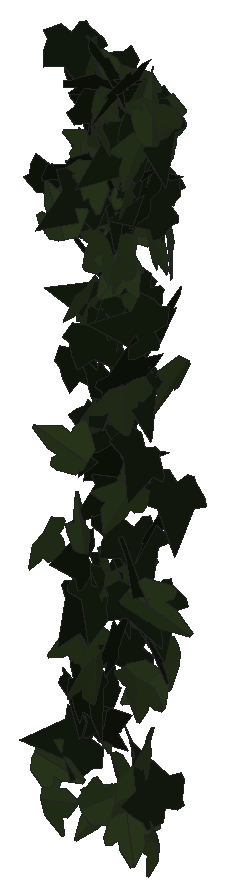
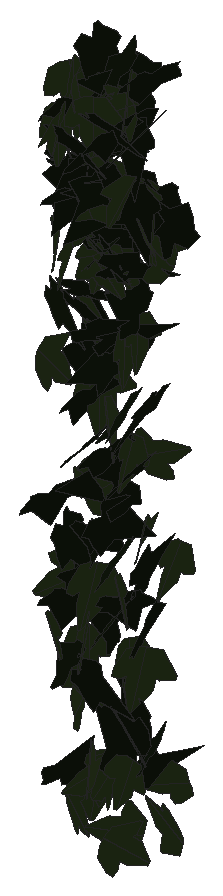
# SketchUp Ruby script. Lengths in inches.
U = 1.inch
M = Sketchup.active_model
def pt(a) = Geom::Point3d.new(a.map { |v| v * U })
def face(e, loops, mat)
  f = e.add_face(loops[0].map { |a| pt(a) })
  loops[1..].each { |l| e.add_face(l.map { |a| pt(a) }).erase! }
  f.material = f.back_material = mat if mat
  f
end
# faces: each face lists its corners as indices into pts; further lists are holes
def faces(e, pts, list, mat = nil) = list.each { |f| face(e, (f[0].is_a?(Array) ? f : [f]).map { |l| l.map { |i| pts[i] } }, mat) }
# xy, xz, yz: faces in a plane at the given z, y or x. An outline is a flat list of corners, or four numbers for a rectangle; further outlines are holes
def ring(l) = l.size == 4 ? [[l[0], l[1]], [l[2], l[1]], [l[2], l[3]], [l[0], l[3]]] : l.each_slice(2).to_a
def flat(e, list, mat, &to3) = list.each { |f| face(e, (f[0].is_a?(Array) ? f : [f]).map { |l| ring(l).map { |u, v| to3.(u, v) } }, mat) }
def xy(e, z, list, mat = nil) = flat(e, list, mat) { |x, y| [x, y, z] }
def xz(e, y, list, mat = nil) = flat(e, list, mat) { |x, z| [x, y, z] }
def yz(e, x, list, mat = nil) = flat(e, list, mat) { |y, z| [x, y, z] }
def lines(e, pts, list) = list.each { |a, b| e.add_line(pt(pts[a]), pt(pts[b])) }
# prism: a flat outline (further loops are holes) pulled along v
def prism(e, loops, v, mat = nil)
  f = face(e, loops, mat); d = Geom::Vector3d.new(v.map { |x| x * U })
  f.pushpull(f.normal.samedirection?(d) ? d.length : -d.length)
end
def box(e, o, s, mat = nil) = prism(e, [[o, [o[0] + s[0], o[1], o[2]], [o[0] + s[0], o[1] + s[1], o[2]], [o[0], o[1] + s[1], o[2]]]], [0, 0, s[2]], mat)
def at(x, y, z, deg = 0) = Geom::Transformation.translation(pt([x, y, z])) * Geom::Transformation.rotation(ORIGIN, Z_AXIS, deg.degrees)
def axes(o, x, y, z) = Geom::Transformation.new([*x, 0, *y, 0, *z, 0, *pt(o).to_a, 1])
def part(name) = M.definitions.add(name)
# library, detail: a bought-in or finely detailed component or shape, given as its bounding box
def library(name, o, s) = part(name).tap { |d| box(d.entities, o, s) }
def detail(e, o, s) = box(e.add_group.entities, o, s)
def put(e, d, t, mat = nil) = e.add_instance(d, t).tap { |i| i.material = mat if mat }
def group(e, t, mat = nil) = e.add_group.tap { |g| g.transformation = t; g.material = mat if mat }.entities
root = M.entities
M.materials.add("efeu1").color = [18, 25, 13]
M.materials.add("efeu2").color = [43, 57, 29]
c1 = part("ivyleaf_10")
p = [[0,0.5,-0.03],[-0.0625,2.02,-0.43],[-0.19,2.01,-0.46],[-0.54,1.05,-0.29],[-0.52,0.625,-0.18],[-0.83,0.76,-0.28],
  [-1.16,0.64,-0.33],[-1.15,0.33,-0.24],[-0.77,-0.39,0.02],[-0.3,-0.51,0.16],[0.04,-0.48,0.23],[-0.02,2.01,-0.4375],
  [-0.06,2.01,-0.43],[0.04,-0.49,0.23],[0.67,-0.49,0.14],[1.38,0.36,-0.2],[1.375,0.51,-0.24],[0.81,0.65,-0.19],
  [0.62,0.59,-0.15],[0.6,1.09,-0.28],[0.5,1.23,-0.31]]
faces(c1.entities,p,[[0,1,2,3,4,5,6,7,8,9,10],[11,12,0,13,14,15,16,17,18,19,20]],"efeu2")
c2 = part("ivyleaf_9")
p = [[1.54,2.16,1.25],[1.36,2.04,1.19],[-0.21,0.99,0.68],[-0.71,1.11,0.82],[-0.85,0.86,0.67],[-0.8,0.17,0.21],
  [-0.9,-0.01,0.1],[-0.67,-0.16,-0.02],[-0.08,-0.08,-0.05],[-0.03,-0.6,-0.4],[0.65,-0.88,-0.66],[0.83,-0.6,-0.49],
  [1.29,-0.42,-0.43],[1.8125,-0.07,-0.26],[1.21,0.44,0.15]]
faces(c2.entities,p,[[0,1,2,3,4,5,6,7,8,9,10,11,12,13,14]],"efeu1")
put(root,c1,axes([564.66,129.125,234.52],[0.19735,-0.83656,0.62727],[-0.15068,0.60893,0.85951],[-1.0347,-0.24823,-0.00552]))
put(root,c1,axes([564.375,130.51,235.96],[0.03234,-0.35529,-0.92496],[0.56311,-0.75489,0.30965],[-0.81529,-0.53548,0.17718]))
put(root,c2,axes([564.27,129.14,235.72],[-0.19011,-0.12223,1.03276],[0.96158,-0.42052,0.12724],[0.39609,0.96223,0.1868]))
put(root,c2,axes([564.42,130.8,241.61],[0.54974,-0.81143,-0.30196],[-0.02082,0.3452,-0.96552],[0.86555,0.52368,0.16856]))
put(root,c1,axes([564.88,128,219.98],[-0.06567,-0.82595,-0.60665],[0.21238,0.58373,-0.81773],[1.00255,-0.17776,0.13349]))
put(root,c2,axes([564.51,130.46,211.35],[0.19359,-0.71401,0.58022],[0.1566,-0.5587,-0.73978],[0.90661,0.24897,0.00389]))
put(root,c2,axes([565.46,130.25,237.87],[0.48085,0.32099,-0.82246],[-0.74029,-0.36372,-0.57477],[-0.48107,0.88054,0.0624]))
put(root,c1,axes([565.57,130.21,237.88],[-0.83667,-0.21288,0.52401],[-0.47896,-0.23101,-0.85858],[0.30084,-0.95981,0.09042]))
put(root,c2,axes([564.84,129.71,228.15],[0.54726,-0.5114,-0.69257],[-0.3479,0.61929,-0.7322],[0.78749,0.62898,0.15782]))
put(root,c1,axes([564.43,128.84,206.97],[0.2933,-0.21869,-1.04088],[0.88147,-0.55426,0.36483],[-0.59521,-0.92858,0.02738]))
put(root,c1,axes([564.55,128.25,209.1875],[0.2406,0.142,0.90249],[0.80852,0.40146,-0.27872],[-0.42539,0.84334,-0.01928]))
put(root,c2,axes([565.66,129.76,209.875],[-0.02498,-0.79926,-0.70561],[-0.01993,-0.70533,0.79965],[-1.06597,0.03192,0.00159]))
put(root,c2,axes([565.4,128.74,237.56],[0.57066,0.82522,-0.07792],[-0.05478,-0.05684,-1.00323],[-0.82708,0.57314,0.01269]))
put(root,c1,axes([565.62,128.08,234.97],[0.88424,0.19811,0.41243],[-0.40106,-0.09632,0.90614],[0.22021,-0.97092,-0.00574]))
put(root,c1,axes([565.42,130.67,210.56],[-0.91603,0.14415,-0.09368],[0.09303,-0.01147,-0.9273],[-0.14457,-0.92074,-0.00312]))
put(root,c2,axes([566.16,130.875,234.49],[-0.73813,-0.23105,0.65374],[-0.59549,-0.27786,-0.77057],[0.35517,-0.94604,0.06666]))
put(root,c2,axes([565.21,129.33,243.39],[0.06529,-0.94013,-0.42619],[0.07375,0.4302,-0.93768],[1.02959,0.0288,0.09419]))
put(root,c1,axes([566.28,128.26,224.28],[0.41224,0.27682,0.93431],[-0.85578,-0.38233,0.49088],[0.46604,-0.94694,0.07493]))
put(root,c1,axes([565.77,129.46,231.25],[0.01711,-0.9549,-0.29214],[0.03731,0.29259,-0.95418],[0.99789,0.00544,0.04069]))
put(root,c1,axes([565.8,129.15,214.99],[-0.68211,-0.81872,-0.27806],[0.18071,0.21137,-1.06562],[0.84555,-0.70563,0.00343]))
put(root,c1,axes([565.88,129.76,225.54],[0.00864,-0.791,-0.58161],[0.08915,0.57986,-0.7873],[0.97775,-0.04588,0.07692]))
put(root,c1,axes([565.74,130.1875,238.24],[0.09132,0.88481,0.46957],[0.01194,0.47053,-0.88892],[-1.00162,0.08628,0.03221]))
put(root,c2,axes([565.67,130.66,224.32],[-0.19662,-0.82672,0.54571],[0.00532,-0.55723,-0.84226],[0.99058,-0.16111,0.11284]))
put(root,c2,axes([565.15,130.36,232.42],[0.47835,-0.53882,0.69882],[0.45037,-0.53449,-0.7204],[0.75884,0.65687,-0.01296]))
put(root,c1,axes([565.98,130.1,230.75],[0.07186,-0.95686,-0.27886],[0.0528,0.28284,-0.95693],[0.99526,0.05408,0.0709]))
put(root,c2,axes([565.96,129.32,218.83],[-0.09449,-0.23298,0.97162],[-0.36011,-0.90242,-0.25141],[0.93201,-0.3723,0.00136]))
put(root,c1,axes([566.2,130.64,206.67],[-0.27259,-0.54875,0.84407],[-0.11609,-0.8515,-0.59107],[1.00006,-0.24842,0.16146]))
put(root,c2,axes([566.3,129.26,236.32],[-0.57538,-0.5983,0.55719],[-0.40314,-0.38512,-0.82985],[0.71127,-0.70228,-0.01961]))
put(root,c2,axes([566.3,129.15,240.3],[0.60577,0.21239,-0.79905],[-0.79349,-0.12896,-0.63584],[-0.23229,0.99439,0.0882]))
put(root,c2,axes([565.625,129.29,216.7],[0.32601,-0.31201,-1.00483],[0.75099,-0.66778,0.45101],[-0.73692,-0.81856,0.01508]))
put(root,c1,axes([566.59,128.95,237.2],[0.61229,-0.02497,-0.8142],[-0.8062,0.12723,-0.61017],[0.11661,1.01076,0.05669]))
put(root,c1,axes([566.23,129.35,242.62],[0.29267,-0.75201,-0.67991],[-0.0384,0.69894,-0.78959],[1.01307,0.24374,0.1665]))
put(root,c1,axes([566.42,128.37,220.19],[-0.2211,0.82835,-0.48441],[-0.18007,0.45246,0.8559],[0.94255,0.28075,0.04988]))
put(root,c2,axes([566.83,130.34,230.6],[-0.4043,-0.76048,-0.65377],[-0.30929,-0.57599,0.86127],[-0.95399,0.50904,-0.00217]))
put(root,c2,axes([566.9,129.33,211.84],[-0.44266,0.65901,0.74542],[-0.40501,0.62587,-0.79382],[-0.9088,-0.59991,-0.00931]))
put(root,c2,axes([566.1875,128.24,213.5],[0.5943,-0.36565,-0.72433],[-0.60709,0.39529,-0.69766],[0.53832,0.84946,0.01287]))
put(root,c2,axes([566.03,131.06,241.12],[0.01227,-1.00353,-0.14543],[-0.01055,0.14531,-1.00357],[1.01396,0.01365,-0.00868]))
put(root,c1,axes([566.74,129.5625,218.35],[0.3735,-0.46335,-0.72167],[-0.41284,0.5928,-0.59427],[0.75171,0.55579,0.0322]))
put(root,c1,axes([566.05,129.69,206.86],[-0.12735,-0.32235,0.95032],[0.3282,0.89188,0.3465],[-0.94832,0.35196,-0.0077]))
put(root,c2,axes([566.91,131.05,241.37],[-0.99688,0.00409,0.06429],[-0.0644,-0.08931,-0.99288],[0.00169,-0.99495,0.08939]))
put(root,c2,axes([566.76,130.97,235.79],[-0.78608,-0.49452,0.32912],[-0.20836,-0.28168,-0.92089],[0.55629,-0.8043,0.12015]))
put(root,c2,axes([566,129.4375,213.25],[-0.37797,-0.16034,-0.92484],[0.9199,0.13495,-0.39935],[0.18662,-0.98994,0.09536]))
put(root,c2,axes([565.99,130.84,217.66],[0.42607,-0.98165,0.06298],[0.02868,-0.05621,-1.07013],[0.98325,0.42702,0.00392]))
put(root,c2,axes([566.03,130.05,227.23],[0.59911,-0.76727,-0.08514],[-0.04238,0.07492,-0.97339],[0.77082,0.60048,0.01266]))
put(root,c1,axes([566,130.11,241.92],[-0.57607,0.12856,-0.81085],[0.69461,-0.45171,-0.5651],[-0.43764,-0.88617,0.17042]))
put(root,c1,axes([566.86,129.16,233.95],[0.79232,-0.30631,-0.63638],[-0.49482,0.44166,-0.82865],[0.50394,0.91525,0.18689]))
put(root,c2,axes([566.78,130.55,222.14],[-0.09942,0.03829,-0.96352],[0.16269,-0.95408,-0.0547],[-0.95046,-0.16732,0.09143]))
put(root,c2,axes([565.76,129.84,210.83],[0.96779,0.04784,-0.53455],[0.51249,0.24487,0.94976],[0.15934,-1.07815,0.19199]))
put(root,c1,axes([566.79,130.83,234.5],[0.81735,0.37506,-0.39642],[-0.37043,-0.14296,-0.89901],[-0.40075,0.89709,0.02247]))
put(root,c2,axes([566.16,130.57,220.16],[0.35934,-0.8808,0.28544],[0.08523,-0.27342,-0.95099],[0.92197,0.36857,-0.02334]))
put(root,c2,axes([566.38,130.82,225.66],[0.02554,-0.93186,-0.28019],[0.02862,0.28089,-0.93156],[0.97265,0.0162,0.03476]))
put(root,c2,axes([566.9,131.45,231.55],[-0.66089,-0.65263,0.2339],[-0.10218,-0.22792,-0.92468],[0.68571,-0.66298,0.08765]))
put(root,c2,axes([566.37,128.91,230.125],[0.39495,-0.62505,-0.72425],[-0.07763,0.76002,-0.69825],[0.95352,0.32077,0.24314]))
put(root,c2,axes([566.75,129.59,217.8],[-0.54492,-0.74016,-0.17178],[0.09337,0.14456,-0.91906],[0.75407,-0.55276,-0.01033]))
put(root,c2,axes([567.66,130.8,214.46],[-0.20538,-0.09178,-1.05774],[-0.9794,-0.39954,0.22484],[-0.40988,1.00068,-0.00725]))
put(root,c1,axes([566.99,131.09,236.58],[-0.53953,-0.76061,0.36563],[0.09575,-0.48633,-0.87041],[0.83848,-0.43389,0.33467]))
put(root,c1,axes([567.49,128.28,240.24],[-0.62458,0.31001,0.74421],[-0.72556,0.19425,-0.68985],[-0.35145,-0.95196,0.10159]))
put(root,c2,axes([566.5625,130.99,235.12],[-0.0708,-0.82447,0.54371],[0.17581,-0.54692,-0.80645],[0.97184,0.03888,0.1855]))
put(root,c1,axes([566.97,130.3125,234.77],[-0.95514,-0.12192,-0.11588],[0.11694,-0.00111,-0.96276],[0.1209,-0.96214,0.0158]))
put(root,c1,axes([567.2,129.72,226.8],[0.38762,-0.90079,-0.45227],[-0.17252,0.41812,-0.98063],[0.99308,0.42424,0.00618]))
put(root,c1,axes([567.17,128.28,214.51],[-0.00092,-1.13497,-0.31256],[0.00662,0.31255,-1.13496],[1.1772,-0.00264,0.00614]))
put(root,c2,axes([566.66,129.43,223.53],[0.0635,0.58103,-0.82301],[0.1299,0.81303,0.58402],[0.99903,-0.14265,-0.02363]))
put(root,c1,axes([567.34,130.71,241.63],[-0.91912,-0.38725,0.12108],[-0.10823,-0.05495,-0.99733],[0.39104,-0.92543,0.00855]))
put(root,c2,axes([566.64,128.84,240.09],[0.00677,-0.02086,1.06759],[0.95023,0.48712,0.00349],[-0.48708,0.95001,0.02165]))
put(root,c2,axes([567.18,129.51,234.13],[-0.66986,0.89332,-0.01825],[-0.01441,0.012,1.11656],[0.89339,0.67,0.00432]))
put(root,c2,axes([566.49,130.36,229.76],[0.88469,-0.52294,0.2093],[0.16965,-0.12423,-1.02749],[0.53712,0.90058,-0.0202]))
put(root,c2,axes([566.48,128.22,241.87],[0.66396,-0.11037,0.7519],[0.72286,0.39986,-0.57962],[-0.23454,0.91994,0.34215]))
put(root,c1,axes([567.23,128.88,241.33],[0.01743,0.78359,0.64214],[-0.21234,0.6308,-0.76398],[-0.99059,-0.12143,0.17507]))
put(root,c2,axes([567.11,129.96,237.09],[0.47654,0.74019,0.50477],[0.18957,0.47548,-0.87621],[-0.87563,0.50576,0.08501]))
put(root,c2,axes([567.1,130.77,235.72],[-0.71374,-0.18844,-0.70116],[0.71407,-0.00441,-0.7257],[0.13128,-1.00051,0.13525]))
put(root,c1,axes([567.88,130.18,222.64],[0.67119,0.03768,0.70919],[-0.70823,-0.03699,0.67224],[0.05277,-0.97574,0.0019]))
put(root,c2,axes([566.89,129.39,242.83],[0.33961,-0.77266,0.60737],[0.34394,-0.50853,-0.83924],[0.92065,0.475,0.08949]))
put(root,c2,axes([567.8,129.83,238.02],[0.38185,0.87653,-0.35288],[-0.18307,-0.30477,-0.95512],[-0.927,0.42126,0.04326]))
put(root,c1,axes([567.32,129.74,209.26],[-0.71277,0.49616,-0.50103],[0.36653,-0.34789,-0.86595],[-0.60237,-0.79878,0.06594]))
put(root,c1,axes([567.85,129.36,233.29],[0.85836,-0.01865,-0.46369],[-0.46257,0.04369,-0.85805],[0.03716,0.97462,0.02959]))
put(root,c1,axes([567.64,129.49,238.08],[-0.80753,-0.55281,-0.28257],[0.23286,0.16006,-0.97863],[0.57552,-0.84044,-0.00051]))
put(root,c1,axes([567.41,130.71,209.25],[-0.52398,0.2867,0.78315],[0.6121,-0.49599,0.59111],[0.56645,0.80118,0.08569]))
put(root,c1,axes([568.07,130.21,216.41],[-0.60922,0.60562,0.52098],[-0.39086,0.34544,-0.85863],[-0.69672,-0.72335,0.02614]))
put(root,c1,axes([567.84,129.86,218.63],[-0.42112,-0.96534,-0.41897],[0.19617,0.37135,-1.05279],[1.03389,-0.46365,0.0291]))
put(root,c2,axes([567.68,130.35,227.83],[0.11097,-0.97649,-0.29116],[0.01919,0.29483,-0.98149],[1.01879,0.10081,0.0502]))
put(root,c2,axes([568.24,127.94,215.44],[0.0147,0.06476,1.01548],[0.25201,0.98371,-0.06638],[-0.98584,0.25244,-0.00183]))
put(root,c1,axes([568.31,128.96,227.62],[-0.44564,-1.10077,-0.12168],[0.03636,0.11655,-1.18752],[1.10688,-0.44701,-0.00998]))
put(root,c2,axes([568.34,130.46,231.89],[-0.91913,-0.08867,-0.348],[0.35135,-0.02419,-0.92181],[0.0743,-0.98251,0.0541]))
put(root,c1,axes([568.46,129.67,231.22],[0.73361,-0.49173,-0.51728],[-0.39484,0.33834,-0.88158],[0.59454,0.83144,0.05281]))
put(root,c2,axes([567.95,129.77,238.91],[0.0879,-0.93191,-0.4056],[-0.03769,0.40384,-0.93605],[1.01565,0.09564,0.00036]))
put(root,c2,axes([568.73,128.875,239.59],[-0.89653,-0.38907,0.27039],[-0.24178,-0.12199,-0.9772],[0.40747,-0.92844,0.01509]))
put(root,c1,axes([568.68,128.67,223.08],[-0.50861,-0.78369,0.47894],[-0.26136,-0.40134,-0.93427],[0.88048,-0.57184,-0.00067]))
put(root,c2,axes([568.76,131.09,240.125],[-1.00709,0.01537,-0.0447],[0.04415,-0.03504,-1.00662],[-0.0169,-1.00747,0.03433]))
put(root,c1,axes([568.45,129.25,237.48],[0.21886,-0.81272,-0.55175],[-0.02353,0.56078,-0.83535],[0.98203,0.19457,0.10295]))
put(root,c1,axes([568.54,130,241.96],[0.23933,-0.98114,-0.10103],[-0.02025,0.09905,-1.00991],[0.98612,0.24016,0.00378]))
put(root,c2,axes([568.1,129.77,220.65],[-0.37769,-0.66772,-0.64977],[0.41911,0.50442,-0.76198],[0.83211,-0.55714,0.08886]))
put(root,c1,axes([568.52,128.41,234.41],[0.20901,-0.71741,-0.74078],[0.15754,0.76919,-0.70047],[1.01912,0.02823,0.26021]))
put(root,c1,axes([568.91,129.94,213.83],[0.76592,0.01934,-0.58414],[-0.58443,0.01621,-0.76577],[-0.00554,0.96311,0.02462]))
put(root,c2,axes([568.78,130.65,220.98],[-0.50352,0.53268,-0.69719],[0.46032,-0.52394,-0.73276],[-0.74694,-0.68197,0.0184]))
put(root,c1,axes([568.7,130.35,234.6],[-0.42271,0.87477,0.34227],[-0.15656,0.30447,-0.97151],[-0.92621,-0.4507,0.00801]))
put(root,c2,axes([568.54,129.625,237.5],[0.64553,0.73783,0.06675],[0.04442,0.04982,-0.98036],[-0.73951,0.64706,-0.00063]))
put(root,c1,axes([568.5,128.6,208.59],[-0.06864,-0.16482,-1.07537],[0.37289,1.00867,-0.1784],[1.02202,-0.37909,-0.00713]))
put(root,c2,axes([568.36,128.71,228.29],[0.6094,0.75277,0.57103],[-0.35334,-0.44863,0.96849],[0.87629,-0.70439,-0.00659]))
put(root,c2,axes([568.33,130.64,237.35],[-0.12945,-0.92337,-0.34098],[0.18456,0.31505,-0.92321],[0.96686,-0.18377,0.13057]))
put(root,c2,axes([569.1,128.29,243.26],[-0.51354,0.70542,-0.56719],[0.18914,-0.55409,-0.86038],[-0.88518,-0.52765,0.14521]))
put(root,c2,axes([568.17,131.1,214.73],[0.23192,-0.68251,0.66954],[0.30761,-0.59906,-0.71722],[0.90525,0.37842,0.07218]))
put(root,c2,axes([568.49,129.9375,224.59],[-0.14579,-0.8937,0.45989],[0.07781,-0.47335,-0.89517],[1.00207,-0.09327,0.13642]))
put(root,c2,axes([568.32,129.73,218.95],[0.05685,-0.55444,0.98982],[0.20117,-0.97043,-0.55513],[1.11655,0.20308,0.04962]))
put(root,c2,axes([568.45,129.33,218.15],[-0.24662,-0.51909,-0.74662],[0.36708,0.65092,-0.57381],[0.83195,-0.44108,0.03186]))
put(root,c2,axes([569.6875,128.8125,237.45],[-0.57319,0.66557,0.53877],[-0.32459,0.43107,-0.87785],[-0.7924,-0.65803,-0.03013]))
put(root,c2,axes([568.74,130.3,217.69],[-0.25288,-0.85343,-0.45675],[0.19473,0.41757,-0.88804],[0.94818,-0.31337,0.06057]))
put(root,c1,axes([568.9,128.36,207.6],[0.58965,0.71891,0.1206],[0.07656,0.09319,-0.9298],[-0.72493,0.5946,-0.0001]))
put(root,c2,axes([569.88,128.74,231.24],[-0.67905,0.26166,0.62516],[-0.66864,-0.11437,-0.67841],[-0.1105,-0.91589,0.26332]))
put(root,c1,axes([569.1,130.78,240.55],[-0.22256,0.96964,-0.12982],[0.00895,-0.13111,-0.99464],[-0.97825,-0.2218,0.02044]))
put(root,c1,axes([569.52,128.31,214.41],[-1.03765,0.08011,0.28638],[-0.28555,0.02176,-1.04074],[-0.08301,-1.07622,0.00027]))
put(root,c1,axes([569.81,128.84,206.8],[0.26573,-0.19376,-1.04021],[-0.7186,0.75419,-0.32406],[0.77666,0.7641,0.05607]))
put(root,c2,axes([569.79,129.61,208.24],[-0.6422,-0.77018,0.1958],[0.14035,0.13786,1.00261],[-0.78219,0.65707,0.01914]))
put(root,c1,axes([569.38,128.52,240.01],[-0.12653,-0.87466,0.44632],[0.13045,-0.461,-0.86643],[0.97325,-0.05192,0.17416]))
put(root,c1,axes([569.21,130.75,234.84],[-0.47162,0.60758,-0.59573],[0.23115,-0.56402,-0.75824],[-0.81891,-0.50912,0.12906]))
put(root,c2,axes([569.15,129.67,240.96],[-0.04173,-0.99592,-0.39194],[0.03331,0.39083,-0.99667],[1.06975,-0.05102,0.01574]))
put(root,c2,axes([569.29,131.12,222.61],[-0.18749,-0.97188,-0.17149],[0.03073,0.16873,-0.9898],[0.98642,-0.18998,-0.00176]))
put(root,c1,axes([569.93,128.9375,241.68],[-0.85499,-0.49771,0.25526],[-0.23565,-0.10234,-0.98887],[0.50729,-0.88639,-0.02916]))
put(root,c2,axes([569.88,130.08,231.61],[-0.74842,0.52503,-0.45128],[0.37413,-0.25245,-0.91419],[-0.58252,-0.83669,-0.00734]))
put(root,c1,axes([569.76,129.89,240.16],[-0.20073,-1.02151,-0.18149],[0.01659,0.18167,-1.04088],[1.03737,-0.20057,-0.01848]))
put(root,c1,axes([569.89,128.57,240.85],[-0.14137,0.99957,-0.54875],[-0.06487,0.545,1.00946],[1.13844,0.15518,-0.01062]))
put(root,c1,axes([569.07,129.11,218.03],[-0.71695,-0.04182,-0.99963],[0.99614,0.08489,-0.718],[0.09334,-1.22722,-0.01561]))
put(root,c2,axes([570.52,129.02,237.24],[-0.86522,0.22294,0.41903],[-0.42737,0.01313,-0.88942],[-0.2065,-0.96126,0.08503]))
put(root,c1,axes([569.59,128.93,211.26],[-0.03085,-0.04989,-0.93839],[0.14735,-0.92754,0.04447],[-0.92809,-0.1456,0.03826]))
put(root,c1,axes([569.97,130.43,228.68],[0.13323,-0.79902,0.62138],[0.06767,-0.61831,-0.80957],[1.00993,0.14684,-0.02773]))
put(root,c1,axes([570.3,129.7,215.45],[0.53811,-0.55875,-0.58439],[-0.39535,0.43051,-0.77566],[0.70528,0.66764,0.01108]))
